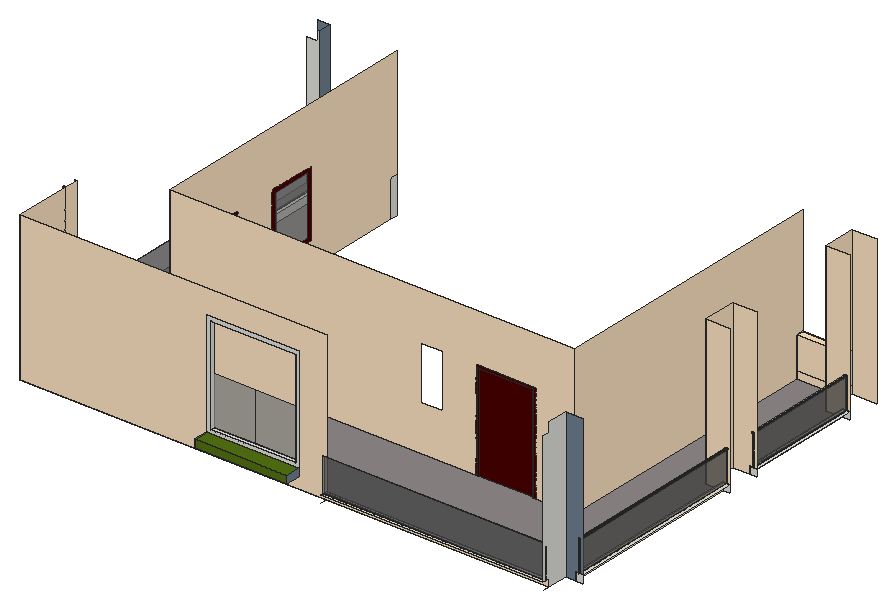
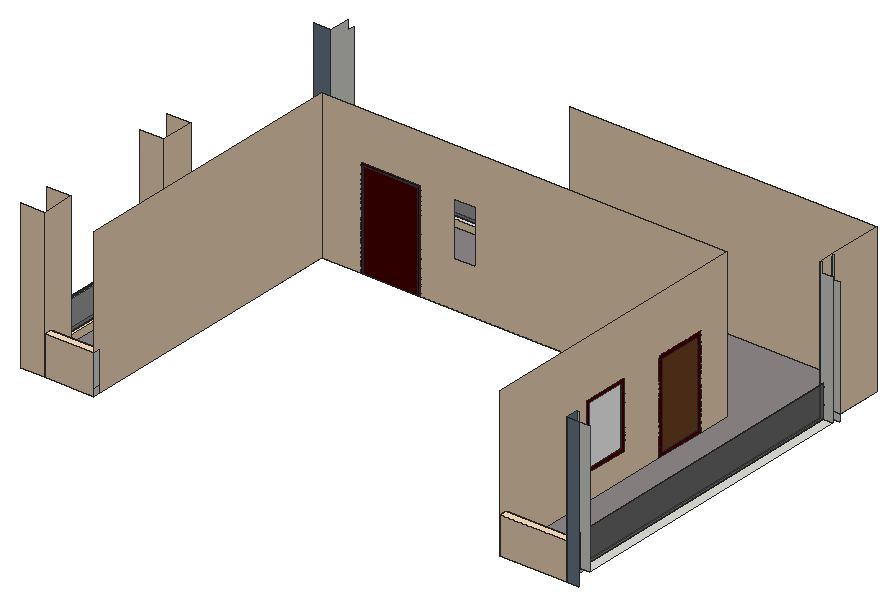
# SketchUp Ruby script. Lengths in inches.
U = 1.inch
M = Sketchup.active_model
def pt(a) = Geom::Point3d.new(a.map { |v| v * U })
def face(e, loops, mat)
  f = e.add_face(loops[0].map { |a| pt(a) })
  loops[1..].each { |l| e.add_face(l.map { |a| pt(a) }).erase! }
  f.material = f.back_material = mat if mat
  f
end
# faces: each face lists its corners as indices into pts; further lists are holes
def faces(e, pts, list, mat = nil) = list.each { |f| face(e, (f[0].is_a?(Array) ? f : [f]).map { |l| l.map { |i| pts[i] } }, mat) }
# xy, xz, yz: faces in a plane at the given z, y or x. An outline is a flat list of corners, or four numbers for a rectangle; further outlines are holes
def ring(l) = l.size == 4 ? [[l[0], l[1]], [l[2], l[1]], [l[2], l[3]], [l[0], l[3]]] : l.each_slice(2).to_a
def flat(e, list, mat, &to3) = list.each { |f| face(e, (f[0].is_a?(Array) ? f : [f]).map { |l| ring(l).map { |u, v| to3.(u, v) } }, mat) }
def xy(e, z, list, mat = nil) = flat(e, list, mat) { |x, y| [x, y, z] }
def xz(e, y, list, mat = nil) = flat(e, list, mat) { |x, z| [x, y, z] }
def yz(e, x, list, mat = nil) = flat(e, list, mat) { |y, z| [x, y, z] }
def lines(e, pts, list) = list.each { |a, b| e.add_line(pt(pts[a]), pt(pts[b])) }
# prism: a flat outline (further loops are holes) pulled along v
def prism(e, loops, v, mat = nil)
  f = face(e, loops, mat); d = Geom::Vector3d.new(v.map { |x| x * U })
  f.pushpull(f.normal.samedirection?(d) ? d.length : -d.length)
end
def box(e, o, s, mat = nil) = prism(e, [[o, [o[0] + s[0], o[1], o[2]], [o[0] + s[0], o[1] + s[1], o[2]], [o[0], o[1] + s[1], o[2]]]], [0, 0, s[2]], mat)
def at(x, y, z, deg = 0) = Geom::Transformation.translation(pt([x, y, z])) * Geom::Transformation.rotation(ORIGIN, Z_AXIS, deg.degrees)
def axes(o, x, y, z) = Geom::Transformation.new([*x, 0, *y, 0, *z, 0, *pt(o).to_a, 1])
def part(name) = M.definitions.add(name)
# library, detail: a bought-in or finely detailed component or shape, given as its bounding box
def library(name, o, s) = part(name).tap { |d| box(d.entities, o, s) }
def detail(e, o, s) = box(e.add_group.entities, o, s)
def put(e, d, t, mat = nil) = e.add_instance(d, t).tap { |i| i.material = mat if mat }
def group(e, t, mat = nil) = e.add_group.tap { |g| g.transformation = t; g.material = mat if mat }.entities
root = M.entities
M.materials.add("[0012_Bisque]").color = [255, 228, 196]
M.materials.add("[0021_DarkRed]").color = [76, 0, 0]
M.materials.add("[0021_DarkRed]1").color = [81, 0, 0]
M.materials.add("[0111_SlateGray]").color = [112, 128, 144]
M.materials.add("[Stone Marble]").color = [143, 138, 136]
M.materials.add("[Translucent Glass Gray]").color = [84, 84, 84]
M.materials["[Translucent Glass Gray]"].alpha = 0.5
M.materials.add("[Translucent Glass Gray]1").color = [128, 128, 128]
M.materials["[Translucent Glass Gray]1"].alpha = 0.5
M.materials.add("[Translucent Resin Crush Gray]").color = [153, 153, 153]
M.materials["[Translucent Resin Crush Gray]"].alpha = 0.8
M.materials.add("[Vegetation Blur 03]").color = [83, 114, 18]
M.materials.add("[Wood Veneer 01]").color = [120, 70, 37]
xy(root,996,[[1584,1366.84,1584,1392,1745,1392,1745,1367.71],[48,1368,264,1392]])
xy(root,996,[[48,132,1767.4375,132,1767.4375,199.52,1800,199.52,1800,798,1745,798,1745,906,1800,906,1800,1284,1745,1284,1745,1367.71,1584,1366.84,1584,468,1446.53,468,1446.53,469.5,1268.41,469.5,1268.41,468,264,468,264,1368,48,1368]],"[Stone Marble]")
xy(root,1008,[[264,587.92,266,733.46]])
xy(root,1020,[[1044,108,1767.4375,118.5],[1044,118.5,1767.4375,120],[1044,120,1767.4375,132],[1812,199.52,1813.5,798],[1813.5,199.52,1824,798],
  [6,360,35.49,1350],[35.49,360,37.49,1350],[37.49,360,48,1350],[1812,906,1814,1284],[1814,906,1824,1284]])
xy(root,1020,[[1800,199.52,1812,798],[1800,906,1812,1284]],"[0012_Bisque]")
xy(root,1057.8,[[683.08,48,983.45,96]],"[0111_SlateGray]")
xy(root,1081.8,[[683.08,48,983.45,96]],"[Vegetation Blur 03]")
xy(root,1088.5,[[264,896.41,266,1029.1875]],"[0021_DarkRed]1")
xy(root,1093.8,[[695.08,96,971.45,108]])
xy(root,1116,[[48,1368,264,1392]],"[0012_Bisque]")
xy(root,1117.8,[[1812,199.52,1813.5,798]])
xy(root,1120.8,[[1812,906,1814,1284]])
xy(root,1123.02,[[1584,1366.84,1745,1367.71,1745,1392,1584,1392]],"[0012_Bisque]")
xz(root,48,[[683.08,1057.8,983.45,1081.8]],"[Vegetation Blur 03]")
xz(root,96,[[[683.08,1081.8,983.45,1423.55],[695.08,1093.8,971.45,1411.55]]])
xz(root,108,[[695.08,1093.8,833.27,1252.68],[833.27,1093.8,971.45,1252.68]],"[Translucent Resin Crush Gray]")
xz(root,118.5,[[1044,1020,1767.4375,1128]],"[Translucent Glass Gray]")
xz(root,120,[[1044,1020,1767.4375,1128]],"[Translucent Glass Gray]")
xz(root,132,[[48,996,48,1476,1044,1476,1044,1020,1767.4375,1020,1767.4375,996]],"[0012_Bisque]")
xz(root,199.52,[[1800,996,1824,1020],[1812,1020,1813.5,1117.8],[1812,1117.8,1812.375,1117.82,1812.75,1117.89,1813.1,1118.01,1813.45,1118.17,1813.76,1118.37,1814.05,1118.61,1814.3125,1118.89,1814.53,1119.19,1814.71,1119.52,1814.85,1119.87,1814.95,1120.24,1814.99,1120.61,1814.99,1120.99,1814.95,1121.36,1814.85,1121.73,1814.71,1122.08,1814.53,1122.41,1814.3125,1122.71,1814.05,1122.99,1813.76,1123.23,1813.45,1123.43,1813.1,1123.59,1812.75,1123.71,1812.375,1123.78,1812,1123.8,1811.625,1123.78,1811.25,1123.71,1810.9,1123.59,1810.55,1123.43,1810.24,1123.23,1809.95,1122.99,1809.6875,1122.71,1809.47,1122.41,1809.29,1122.08,1809.15,1121.73,1809.05,1121.36,1809.01,1120.99,1809.01,1120.61,1809.05,1120.24,1809.15,1119.87,1809.29,1119.52,1809.47,1119.19,1809.6875,1118.89,1809.95,1118.61,1810.24,1118.37,1810.55,1118.17,1810.9,1118.01,1811.25,1117.89,1811.625,1117.82]])
xz(root,199.52,[[[1767.4375,996,1767.4375,1476,1824,1476,1824,1020,1800,1020,1800,996],[1812,1117.8,1812.375,1117.82,1812.75,1117.89,1813.1,1118.01,1813.45,1118.17,1813.76,1118.37,1814.05,1118.61,1814.3125,1118.89,1814.53,1119.19,1814.71,1119.52,1814.85,1119.87,1814.95,1120.24,1814.99,1120.61,1814.99,1120.99,1814.95,1121.36,1814.85,1121.73,1814.71,1122.08,1814.53,1122.41,1814.3125,1122.71,1814.05,1122.99,1813.76,1123.23,1813.45,1123.43,1813.1,1123.59,1812.75,1123.71,1812.375,1123.78,1812,1123.8,1811.625,1123.78,1811.25,1123.71,1810.9,1123.59,1810.55,1123.43,1810.24,1123.23,1809.95,1122.99,1809.6875,1122.71,1809.47,1122.41,1809.29,1122.08,1809.15,1121.73,1809.05,1121.36,1809.01,1120.99,1809.01,1120.61,1809.05,1120.24,1809.15,1119.87,1809.29,1119.52,1809.47,1119.19,1809.6875,1118.89,1809.95,1118.61,1810.24,1118.37,1810.55,1118.17,1810.9,1118.01,1811.25,1117.89,1811.625,1117.82]]],"[0111_SlateGray]")
xz(root,312,[[24,996,48,1020],[24,1020,48,1020,48,1476,42,1476,42,1404,24,1404]])
xz(root,360,[[[6,1020,6,1445.3125,42,1445.3125,42,1476,48,1476,48,1020],[37.18,1125.02,37.49,1125.03,37.81,1125.02,38.12,1125.07,38.42,1125.15,38.71,1125.26,38.99,1125.4,39.26,1125.57,39.5,1125.77,39.72,1125.99,39.92,1126.24,40.09,1126.5,40.24,1126.78,40.35,1127.07,40.43,1127.375,40.48,1127.6875,40.49,1128,40.48,1128.3125,40.43,1128.625,40.35,1128.93,40.24,1129.22,40.09,1129.5,39.92,1129.76,39.72,1130.01,39.5,1130.23,39.26,1130.43,38.99,1130.6,38.71,1130.74,38.42,1130.85,38.12,1130.93,37.81,1130.98,37.49,1131,37.18,1130.98,36.87,1130.93,36.57,1130.85,36.27,1130.74,35.99,1130.6,35.73,1130.43,35.49,1130.23,35.26,1130.01,35.07,1129.76,34.9,1129.5,34.75,1129.22,34.64,1128.93,34.56,1128.625,34.51,1128.3125,34.49,1128,34.51,1127.6875,34.56,1127.375,34.64,1127.07,34.75,1126.78,34.9,1126.5,35.07,1126.24,35.26,1125.99,35.49,1125.77,35.73,1125.57,35.99,1125.4,36.27,1125.26,36.57,1125.15,36.87,1125.07,37.125,1125.03]],[35.49,1020,37.49,1020,37.49,1125.03,37.18,1125.02,37.125,1125.03,35.49,1125.03]])
xz(root,468,[[[264,996,1260.41,996,1260.41,1319.1875,1454.53,1319.1875,1454.53,996,1584,996,1584,1476,264,1476],[1080.18,1144.0625,1153.12,1319.1875]]],"[0012_Bisque]")
xz(root,468,[[1260.41,996,1268.41,996,1268.41,1311.1875,1446.53,1311.1875,1446.53,996,1454.53,996,1454.53,1319.1875,1260.41,1319.1875]],"[0021_DarkRed]")
xz(root,469.5,[[1268.41,996,1446.53,1311.1875]],"[0021_DarkRed]")
xz(root,587.92,[[264,1008,266,1281.1]])
xz(root,733.46,[[264,1008,266,1281.1]],"[0021_DarkRed]1")
xz(root,798,[[1800,996,1824,1020],[1812,1020,1813.5,1117.8]])
xz(root,798,[[[1745,996,1800,996,1800,1020,1824,1020,1824,1476,1745,1476],[1812,1117.8,1811.625,1117.82,1811.25,1117.89,1810.9,1118.01,1810.55,1118.17,1810.24,1118.37,1809.95,1118.61,1809.6875,1118.89,1809.47,1119.19,1809.29,1119.52,1809.15,1119.87,1809.05,1120.24,1809.01,1120.61,1809.01,1120.99,1809.05,1121.36,1809.15,1121.73,1809.29,1122.08,1809.47,1122.41,1809.6875,1122.71,1809.95,1122.99,1810.24,1123.23,1810.55,1123.43,1810.9,1123.59,1811.25,1123.71,1811.625,1123.78,1812,1123.8,1812.375,1123.78,1812.75,1123.71,1813.1,1123.59,1813.45,1123.43,1813.76,1123.23,1814.05,1122.99,1814.3125,1122.71,1814.53,1122.41,1814.71,1122.08,1814.85,1121.73,1814.95,1121.36,1814.99,1120.99,1814.99,1120.61,1814.95,1120.24,1814.85,1119.87,1814.71,1119.52,1814.53,1119.19,1814.3125,1118.89,1814.05,1118.61,1813.76,1118.37,1813.45,1118.17,1813.1,1118.01,1812.75,1117.89,1812.375,1117.82]]],"[0012_Bisque]")
xz(root,896.41,[[264,1088.5,266,1281.1]])
xz(root,906,[[1800,996,1824,1020],[1812,1020,1814,1020,1814,1117.82,1812.21,1117.82,1812.14,1117.8,1812,1117.82],[1812.14,1117.8,1812.21,1117.82,1812,1117.82],[1812,1117.82,1812.21,1117.82,1812.91,1117.94,1813.62,1118.28,1814,1118.6,1814,1120.8,1812,1120.8],[1812.21,1117.82,1814,1117.82,1814,1118.6,1813.62,1118.28,1812.91,1117.94]])
xz(root,906,[[[1745,996,1745,1476,1824,1476,1824,1020,1800,1020,1800,996],[1812.14,1117.8,1812.21,1117.82,1812.91,1117.94,1813.62,1118.28,1814,1118.6,1814.22,1118.78,1814.67,1119.42,1814.93,1120.16,1815,1120.94,1814.86,1121.71,1814.52,1122.42,1814.02,1123.02,1813.375,1123.47,1812.64,1123.73,1811.86,1123.8,1811.09,1123.66,1810.38,1123.32,1809.78,1122.82,1809.33,1122.18,1809.07,1121.44,1809,1120.66,1809.14,1119.89,1809.48,1119.18,1809.98,1118.58,1810.625,1118.13,1811.36,1117.87,1812,1117.82]]],"[0012_Bisque]")
xz(root,1029.1875,[[264,1088.5,266,1281.1]],"[0021_DarkRed]1")
xz(root,1284,[[1800,996,1824,1020],[1812,1020,1812,1117.82,1812.14,1117.8,1812.21,1117.82,1814,1117.82,1814,1020],[1812.14,1117.8,1812,1117.82,1812.21,1117.82],[1812,1117.82,1811.36,1117.87,1810.625,1118.13,1809.98,1118.58,1809.48,1119.18,1809.14,1119.89,1809,1120.66,1809.07,1121.44,1809.33,1122.18,1809.78,1122.82,1810.38,1123.32,1811.09,1123.66,1811.86,1123.8,1812.64,1123.73,1813.375,1123.47,1814.02,1123.02,1814.52,1122.42,1814.86,1121.71,1815,1120.94,1814.93,1120.16,1814.67,1119.42,1814.22,1118.78,1814,1118.6,1814,1120.8,1812,1120.8],[1812,1117.82,1812,1120.8,1814,1120.8,1814,1118.6,1813.62,1118.28,1812.91,1117.94,1812.21,1117.82],
  [1812.21,1117.82,1812.91,1117.94,1813.62,1118.28,1814,1118.6,1814,1117.82]])
xz(root,1284,[[[1745,996,1800,996,1800,1020,1824,1020,1824,1476,1745,1476],[1812.14,1117.8,1812,1117.82,1811.36,1117.87,1810.625,1118.13,1809.98,1118.58,1809.48,1119.18,1809.14,1119.89,1809,1120.66,1809.07,1121.44,1809.33,1122.18,1809.78,1122.82,1810.38,1123.32,1811.09,1123.66,1811.86,1123.8,1812.64,1123.73,1813.375,1123.47,1814.02,1123.02,1814.52,1122.42,1814.86,1121.71,1815,1120.94,1814.93,1120.16,1814.67,1119.42,1814.22,1118.78,1814,1118.6,1813.62,1118.28,1812.91,1117.94,1812.21,1117.82]]],"[0012_Bisque]")
xz(root,1350,[[[6,1020,48,1020,48,1476,42,1476,42,1445.3125,6,1445.3125],[37.18,1125.02,37.125,1125.03,36.87,1125.07,36.57,1125.15,36.27,1125.26,35.99,1125.4,35.73,1125.57,35.49,1125.77,35.26,1125.99,35.07,1126.24,34.9,1126.5,34.75,1126.78,34.64,1127.07,34.56,1127.375,34.51,1127.6875,34.49,1128,34.51,1128.3125,34.56,1128.625,34.64,1128.93,34.75,1129.22,34.9,1129.5,35.07,1129.76,35.26,1130.01,35.49,1130.23,35.73,1130.43,35.99,1130.6,36.27,1130.74,36.57,1130.85,36.87,1130.93,37.18,1130.98,37.49,1131,37.81,1130.98,38.12,1130.93,38.42,1130.85,38.71,1130.74,38.99,1130.6,39.26,1130.43,39.5,1130.23,39.72,1130.01,39.92,1129.76,40.09,1129.5,40.24,1129.22,40.35,1128.93,40.43,1128.625,40.48,1128.3125,40.49,1128,40.48,1127.6875,40.43,1127.375,40.35,1127.07,40.24,1126.78,40.09,1126.5,39.92,1126.24,39.72,1125.99,39.5,1125.77,39.26,1125.57,38.99,1125.4,38.71,1125.26,38.42,1125.15,38.12,1125.07,37.81,1125.02,37.49,1125.03]],[35.49,1020,35.49,1125.03,37.125,1125.03,37.18,1125.02,37.49,1125.03,37.49,1020]])
xz(root,1368,[[48,996,264,1116]],"[0012_Bisque]")
xz(root,1392,[[48,996,264,1116],[1584,996,1745,1123.02],[1745,996,1824,1476]],"[0012_Bisque]")
xz(root,1392,[[6,996,48,1476]],"[0111_SlateGray]")
yz(root,35.49,[[360,1020,1350,1125.03]],"[Translucent Glass Gray]")
yz(root,37.49,[[360,1020,1350,1125.03]],"[Translucent Glass Gray]")
yz(root,48,[[312,996,1368,1020],[1368,996,1392,1020],[1350,1020,1368,1116],[1368,1020,1392,1116]])
yz(root,48,[[132,996,312,1476],[312,1020,360,1476]],"[0012_Bisque]")
yz(root,48,[[1350,1116,1392,1476]],"[0111_SlateGray]")
yz(root,264,[[1368,996,1392,1116]])
yz(root,264,[[[468,996,468,1476,1392,1476,1392,1116,1368,1116,1368,996,745.46,996,745.46,1293.1,575.92,1293.1,575.92,996],[884.41,1076.5,1041.1875,1293.1]]],"[0012_Bisque]")
yz(root,264,[[[575.92,996,745.46,1293.1],[587.92,1008,733.46,1281.1]],[[884.41,1076.5,1041.1875,1293.1],[896.41,1088.5,1029.1875,1281.1]]],"[0021_DarkRed]1")
yz(root,266,[[896.41,1088.5,1029.1875,1281.1]],"[Translucent Glass Gray]1")
yz(root,266,[[587.92,1008,733.46,1281.1]],"[Wood Veneer 01]")
yz(root,683.08,[[48,1057.8,96,1081.8]],"[0111_SlateGray]")
yz(root,695.08,[[96,1093.8,108,1411.55]])
yz(root,971.45,[[96,1093.8,108,1411.55]])
yz(root,983.45,[[48,1057.8,96,1081.8]],"[0111_SlateGray]")
yz(root,1044,[[118.5,1020,120,1125.02]])
yz(root,1268.41,[[468,996,469.5,1311.1875]],"[0021_DarkRed]")
yz(root,1446.53,[[468,996,469.5,1311.1875]],"[0021_DarkRed]")
yz(root,1584,[[1366.84,996,1392,1020],[1366.84,1020,1392,1123.02]])
yz(root,1584,[[468,996,1366.84,996,1366.84,1123.02,1392,1123.02,1392,1476,468,1476]],"[0012_Bisque]")
yz(root,1745,[[1367.71,996,1392,1020],[1367.71,1020,1392,1123.02]])
yz(root,1745,[[798,996,906,1476],[1284,996,1284,1476,1392,1476,1392,1123.02,1367.71,1123.02,1367.71,996]],"[0012_Bisque]")
yz(root,1767.4375,[[[132,996,132,1020,108,1020,108,1446,132,1446,132,1476,199.52,1476,199.52,996],[120,1125.02,120.3125,1125.02,121.08,1125.2,121.76,1125.57,122.33,1126.11,122.74,1126.78,122.96,1127.53,122.98,1128.3125,122.8,1129.08,122.43,1129.76,121.89,1130.33,121.22,1130.74,120.47,1130.96,119.6875,1130.98,118.92,1130.8,118.24,1130.43,117.67,1129.89,117.26,1129.22,117.04,1128.47,117.02,1127.6875,117.2,1126.92,117.57,1126.24,118.11,1125.67,118.5,1125.43,118.78,1125.26,119.53,1125.04]],[118.5,1020,120,1125.02]])
yz(root,1800,[[199.52,996,798,1020],[906,996,1284,1020]],"[0012_Bisque]")
yz(root,1809.01,[[199.52,1120.61,798,1120.99]])
yz(root,1812,[[199.52,1117.8,798,1120.8]])
yz(root,1812,[[199.52,1020,798,1117.8],[906,1020,1284,1120.8]],"[Translucent Glass Gray]")
yz(root,1813.5,[[199.52,1020,798,1117.8]],"[Translucent Glass Gray]")
yz(root,1814,[[906,1020,1284,1120.8]],"[Translucent Glass Gray]")
yz(root,1814.99,[[199.52,1120.61,798,1120.99]])
p = [[1584,1366.84,996],[1745,1367.71,996],[1745,1367.71,1020],[1584,1366.84,1020],[1745,1367.71,1123.02],[1584,1366.84,1123.02],
  [1811.625,199.52,1117.82],[1811.25,199.52,1117.89],[1811.25,798,1117.89],[1811.625,798,1117.82],[1812,199.52,1117.8],[1812,798,1117.8],
  [1812.375,199.52,1117.82],[1812.375,798,1117.82],[1812.75,199.52,1117.89],[1812.75,798,1117.89],[1811.36,1284,1117.87],[1812,1284,1117.82],
  [1812.14,1284,1117.8],[1812.14,906,1117.8],[1812,906,1117.82],[1811.36,906,1117.87],[1812.21,1284,1117.82],[1812.91,1284,1117.94],
  [1812.91,906,1117.94],[1812.21,906,1117.82],[1810.9,199.52,1118.01],[1810.9,798,1118.01],[1813.1,199.52,1118.01],[1813.1,798,1118.01],
  [1810.625,1284,1118.13],[1810.625,906,1118.13],[1813.62,1284,1118.28],[1813.62,906,1118.28],[1810.55,199.52,1118.17],[1810.55,798,1118.17],
  [1813.45,199.52,1118.17],[1813.45,798,1118.17],[1809.98,1284,1118.58],[1809.98,906,1118.58],[1810.24,199.52,1118.37],[1810.24,798,1118.37],
  [1813.76,199.52,1118.37],[1813.76,798,1118.37],[1814,1284,1118.6],[1814.22,1284,1118.78],[1814.22,906,1118.78],[1814,906,1118.6],
  [1809.95,199.52,1118.61],[1809.95,798,1118.61],[1814.05,199.52,1118.61],[1814.05,798,1118.61],[1809.6875,199.52,1118.89],[1809.6875,798,1118.89],
  [1814.3125,199.52,1118.89],[1814.3125,798,1118.89],[1809.48,1284,1119.18],[1809.48,906,1119.18],[1814.67,1284,1119.42],[1814.67,906,1119.42],
  [1809.47,199.52,1119.19],[1809.47,798,1119.19],[1814.53,199.52,1119.19],[1814.53,798,1119.19],[1809.29,199.52,1119.52],[1809.29,798,1119.52],
  [1814.71,199.52,1119.52],[1814.71,798,1119.52],[1809.14,1284,1119.89],[1809.14,906,1119.89],[1814.93,1284,1120.16],[1814.93,906,1120.16],
  [1809.15,199.52,1119.87],[1809.15,798,1119.87],[1814.85,199.52,1119.87],[1814.85,798,1119.87],[1809.05,199.52,1120.24],[1809.05,798,1120.24],
  [1814.95,199.52,1120.24],[1814.95,798,1120.24],[1809,1284,1120.66],[1809,906,1120.66],[1809.01,199.52,1120.61],[1809.01,798,1120.61],
  [1814.99,199.52,1120.61],[1814.99,798,1120.61],[1815,1284,1120.94],[1815,906,1120.94],[1809.07,1284,1121.44],[1809.07,906,1121.44],
  [1814.86,1284,1121.71],[1814.86,906,1121.71],[1809.01,199.52,1120.99],[1809.05,199.52,1121.36],[1809.05,798,1121.36],[1809.01,798,1120.99],
  [1814.95,199.52,1121.36],[1814.99,199.52,1120.99],[1814.99,798,1120.99],[1814.95,798,1121.36],[1809.15,199.52,1121.73],[1809.15,798,1121.73],
  [1814.85,199.52,1121.73],[1814.85,798,1121.73],[1809.33,1284,1122.18],[1809.33,906,1122.18],[1809.29,199.52,1122.08],[1809.29,798,1122.08],
  [1814.71,199.52,1122.08],[1814.71,798,1122.08],[1814.52,1284,1122.42],[1814.52,906,1122.42],[1809.47,199.52,1122.41],[1809.47,798,1122.41],
  [1814.53,199.52,1122.41],[1814.53,798,1122.41],[1809.78,1284,1122.82],[1809.78,906,1122.82],[1809.6875,199.52,1122.71],[1809.6875,798,1122.71],
  [1814.3125,199.52,1122.71],[1814.3125,798,1122.71],[1814.02,1284,1123.02],[1814.02,906,1123.02],[1809.95,199.52,1122.99],[1809.95,798,1122.99],
  [1814.05,199.52,1122.99],[1814.05,798,1122.99],[1810.38,1284,1123.32],[1810.38,906,1123.32],[1810.24,199.52,1123.23],[1810.24,798,1123.23],
  [1813.76,199.52,1123.23],[1813.76,798,1123.23],[1813.375,1284,1123.47],[1813.375,906,1123.47],[1810.55,199.52,1123.43],[1810.55,798,1123.43],
  [1813.45,199.52,1123.43],[1813.45,798,1123.43],[1811.09,1284,1123.66],[1811.09,906,1123.66],[1810.9,199.52,1123.59],[1810.9,798,1123.59],
  [1813.1,199.52,1123.59],[1813.1,798,1123.59],[1812.64,1284,1123.73],[1812.64,906,1123.73],[1811.25,199.52,1123.71],[1811.25,798,1123.71],
  [1812.75,199.52,1123.71],[1812.75,798,1123.71],[1811.625,199.52,1123.78],[1811.625,798,1123.78],[1812.375,199.52,1123.78],[1812.375,798,1123.78],
  [1811.86,1284,1123.8],[1811.86,906,1123.8],[1812,199.52,1123.8],[1812,798,1123.8],[1044,108,996],[1044,132,996],
  [1767.4375,132,996],[1767.4375,108,996]]
faces(root,p,[[0,1,2,3],[3,2,4,5]],"[0012_Bisque]")
faces(root,p,[[6,7,8,9],[10,6,9,11],[12,10,11,13],[14,12,13,15],[16,17,18,19,20,21],[18,22,23,24,25,19],[7,26,27,8],[28,14,15,29],
  [30,16,21,31],[23,32,33,24],[26,34,35,27],[36,28,29,37],[38,30,31,39],[34,40,41,35],[42,36,37,43],[32,44,45,46,47,33],
  [40,48,49,41],[50,42,43,51],[48,52,53,49],[54,50,51,55],[56,38,39,57],[45,58,59,46],[52,60,61,53],[62,54,55,63],
  [60,64,65,61],[66,62,63,67],[68,56,57,69],[58,70,71,59],[64,72,73,65],[74,66,67,75],[72,76,77,73],[78,74,75,79],
  [80,68,69,81],[76,82,83,77],[84,78,79,85],[70,86,87,71],[88,80,81,89],[86,90,91,87],[92,93,94,95],[96,97,98,99],
  [93,100,101,94],[102,96,99,103],[104,88,89,105],[100,106,107,101],[108,102,103,109],[90,110,111,91],[106,112,113,107],[114,108,109,115],
  [116,104,105,117],[112,118,119,113],[120,114,115,121],[110,122,123,111],[118,124,125,119],[126,120,121,127],[128,116,117,129],[124,130,131,125],
  [132,126,127,133],[122,134,135,123],[130,136,137,131],[138,132,133,139],[140,128,129,141],[136,142,143,137],[144,138,139,145],[134,146,147,135],
  [142,148,149,143],[150,144,145,151],[148,152,153,149],[154,150,151,155],[156,140,141,157],[146,156,157,147],[152,158,159,153],[158,154,155,159]])
lines(root,p,[[160,161],[162,163]])
